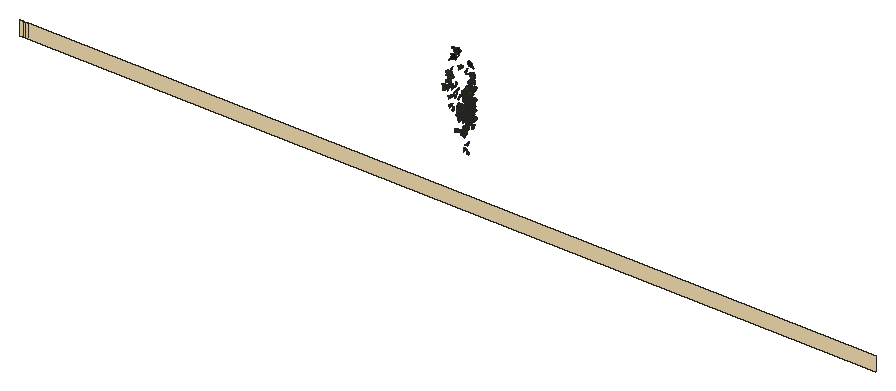
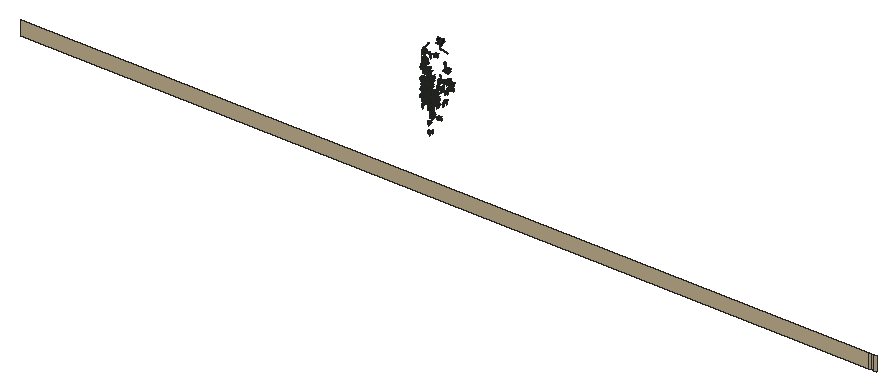
# SketchUp Ruby script. Lengths in inches.
U = 1.inch
M = Sketchup.active_model
def pt(a) = Geom::Point3d.new(a.map { |v| v * U })
def face(e, loops, mat)
  f = e.add_face(loops[0].map { |a| pt(a) })
  loops[1..].each { |l| e.add_face(l.map { |a| pt(a) }).erase! }
  f.material = f.back_material = mat if mat
  f
end
# faces: each face lists its corners as indices into pts; further lists are holes
def faces(e, pts, list, mat = nil) = list.each { |f| face(e, (f[0].is_a?(Array) ? f : [f]).map { |l| l.map { |i| pts[i] } }, mat) }
# xy, xz, yz: faces in a plane at the given z, y or x. An outline is a flat list of corners, or four numbers for a rectangle; further outlines are holes
def ring(l) = l.size == 4 ? [[l[0], l[1]], [l[2], l[1]], [l[2], l[3]], [l[0], l[3]]] : l.each_slice(2).to_a
def flat(e, list, mat, &to3) = list.each { |f| face(e, (f[0].is_a?(Array) ? f : [f]).map { |l| ring(l).map { |u, v| to3.(u, v) } }, mat) }
def xy(e, z, list, mat = nil) = flat(e, list, mat) { |x, y| [x, y, z] }
def xz(e, y, list, mat = nil) = flat(e, list, mat) { |x, z| [x, y, z] }
def yz(e, x, list, mat = nil) = flat(e, list, mat) { |y, z| [x, y, z] }
def lines(e, pts, list) = list.each { |a, b| e.add_line(pt(pts[a]), pt(pts[b])) }
# prism: a flat outline (further loops are holes) pulled along v
def prism(e, loops, v, mat = nil)
  f = face(e, loops, mat); d = Geom::Vector3d.new(v.map { |x| x * U })
  f.pushpull(f.normal.samedirection?(d) ? d.length : -d.length)
end
def box(e, o, s, mat = nil) = prism(e, [[o, [o[0] + s[0], o[1], o[2]], [o[0] + s[0], o[1] + s[1], o[2]], [o[0], o[1] + s[1], o[2]]]], [0, 0, s[2]], mat)
def at(x, y, z, deg = 0) = Geom::Transformation.translation(pt([x, y, z])) * Geom::Transformation.rotation(ORIGIN, Z_AXIS, deg.degrees)
def axes(o, x, y, z) = Geom::Transformation.new([*x, 0, *y, 0, *z, 0, *pt(o).to_a, 1])
def part(name) = M.definitions.add(name)
# library, detail: a bought-in or finely detailed component or shape, given as its bounding box
def library(name, o, s) = part(name).tap { |d| box(d.entities, o, s) }
def detail(e, o, s) = box(e.add_group.entities, o, s)
def put(e, d, t, mat = nil) = e.add_instance(d, t).tap { |i| i.material = mat if mat }
def group(e, t, mat = nil) = e.add_group.tap { |g| g.transformation = t; g.material = mat if mat }.entities
root = M.entities
M.materials.add("1026 AP 7946 SUNNY SIDE UP").color = [254, 231, 186]
M.materials.add("efeu1").color = [18, 25, 13]
M.materials.add("efeu2").color = [43, 57, 29]
c1 = part("ivyleaf_10")
p = [[0,0.5,-0.03],[-0.0625,2.02,-0.43],[-0.19,2.01,-0.46],[-0.54,1.05,-0.29],[-0.52,0.625,-0.18],[-0.83,0.76,-0.28],
  [-1.16,0.64,-0.33],[-1.15,0.33,-0.24],[-0.77,-0.39,0.02],[-0.3,-0.51,0.16],[0.04,-0.48,0.23],[-0.02,2.01,-0.4375],
  [-0.06,2.01,-0.43],[0.04,-0.49,0.23],[0.67,-0.49,0.14],[1.38,0.36,-0.2],[1.375,0.51,-0.24],[0.81,0.65,-0.19],
  [0.62,0.59,-0.15],[0.6,1.09,-0.28],[0.5,1.23,-0.31]]
faces(c1.entities,p,[[0,1,2,3,4,5,6,7,8,9,10],[11,12,0,13,14,15,16,17,18,19,20]],"efeu2")
c2 = part("ivyleaf_9")
p = [[1.54,2.16,1.25],[1.36,2.04,1.19],[-0.21,0.99,0.68],[-0.71,1.11,0.82],[-0.85,0.86,0.67],[-0.8,0.17,0.21],
  [-0.9,-0.01,0.1],[-0.67,-0.16,-0.02],[-0.08,-0.08,-0.05],[-0.03,-0.6,-0.4],[0.65,-0.88,-0.66],[0.83,-0.6,-0.49],
  [1.29,-0.42,-0.43],[1.8125,-0.07,-0.26],[1.21,0.44,0.15]]
faces(c2.entities,p,[[0,1,2,3,4,5,6,7,8,9,10,11,12,13,14]],"efeu1")
xz(root,213.1,[[29.49,246,29.75,248],[29.75,246,152.98,248]],"1026 AP 7946 SUNNY SIDE UP")
p = [[28.98,213.12,246],[28.98,213.12,248],[28.65,213.13,248],[28.65,213.13,246],[29.19,213.11,246],[29.19,213.11,248],
  [29.49,213.1,246],[29.49,213.1,248]]
faces(root,p,[[0,1,2,3],[4,5,1,0],[6,7,5,4]],"1026 AP 7946 SUNNY SIDE UP")
put(root,c1,axes([90.43,213.11,261.01],[0.21131,0.11138,-0.12925],[-0.15052,-0.08209,-0.18028],[-0.21754,0.16498,-0.00081]),"1026 AP 7946 SUNNY SIDE UP")
put(root,c1,axes([90.74,212.72,261.5625],[-0.28486,-0.07479,0.10189],[-0.1113,-0.08227,-0.1973],[0.16073,-0.18952,0.04395]),"1026 AP 7946 SUNNY SIDE UP")
put(root,c1,axes([90.68,213.08,261.15],[0.03809,0.2156,-0.007],[-0.00257,-0.00789,-0.22355],[-0.33923,0.02427,0.00091]),"1026 AP 7946 SUNNY SIDE UP")
put(root,c1,axes([90.82,213.05,262.11],[-0.11033,-0.17291,-0.12471],[0.18767,0.07159,-0.17763],[0.27267,-0.11923,0.0718]),"1026 AP 7946 SUNNY SIDE UP")
put(root,c1,axes([91.14,212.875,263.34],[0.33201,0.02527,-0.08737],[-0.12701,-0.03553,-0.2179],[-0.05739,0.22481,-0.02325]),"1026 AP 7946 SUNNY SIDE UP")
put(root,c1,axes([91.26,213,261.64],[-0.11322,-0.2058,0.02896],[-0.00445,-0.03002,-0.22467],[0.32683,-0.0717,0.00698]),"1026 AP 7946 SUNNY SIDE UP")
put(root,c1,axes([91.27,212.99,260.25],[-0.06266,-0.17143,0.12102],[0.02951,-0.12305,-0.1777],[0.32631,-0.02179,0.03931]),"1026 AP 7946 SUNNY SIDE UP")
put(root,c1,axes([91.35,213.01,259.1],[-0.02837,-0.19808,0.05526],[0.00033,-0.055,-0.20517],[0.32315,-0.01733,0.00506]),"1026 AP 7946 SUNNY SIDE UP")
put(root,c1,axes([91.35,212.87,262.98],[0.33522,0.0503,-0.06781],[-0.09987,-0.01866,-0.22574],[-0.08419,0.22242,-0.00223]),"1026 AP 7946 SUNNY SIDE UP")
put(root,c1,axes([91.45,212.98,263.93],[0.10871,-0.22409,0.02547],[0.00264,-0.02667,-0.24167],[0.35472,0.06887,-0.00601]),"1026 AP 7946 SUNNY SIDE UP")
put(root,c1,axes([91.64,212.99,261.61],[-0.10015,-0.2016,0.0619],[0.00589,-0.06504,-0.21697],[0.33123,-0.0598,0.02258]),"1026 AP 7946 SUNNY SIDE UP")
put(root,c1,axes([91.59,213,258.76],[0.05866,-0.19159,-0.06292],[0.04007,0.06504,-0.19729],[0.31313,0.02757,0.03704]),"1026 AP 7946 SUNNY SIDE UP")
put(root,c1,axes([91.74,213,260.67],[0.12014,-0.20112,-0.00474],[-0.00381,0.00278,-0.22162],[0.31627,0.07643,-0.00087]),"1026 AP 7946 SUNNY SIDE UP")
put(root,c2,axes([91.9,212.98,265.61],[-0.38272,0.01155,-0.00637],[0.00608,-0.04787,-0.24647],[-0.01974,-0.23873,0.04766]),"1026 AP 7946 SUNNY SIDE UP")
put(root,c1,axes([92.04,213.01,262.04],[0.13694,-0.18694,-0.08959],[-0.03553,0.08402,-0.21149],[0.32153,0.0889,0.01479]),"1026 AP 7946 SUNNY SIDE UP")
put(root,c1,axes([92.04,213,260.51],[0.04944,-0.20726,-0.04746],[-0.01887,0.04357,-0.21564],[0.33291,0.03325,-0.00517]),"1026 AP 7946 SUNNY SIDE UP")
put(root,c2,axes([92.06,212.86,266.8],[0.28129,0.11124,-0.138],[-0.16928,-0.08143,-0.21723],[-0.21616,0.20853,-0.00946]),"1026 AP 7946 SUNNY SIDE UP")
put(root,c1,axes([92.11,213,266.48],[0.29158,0.16408,-0.0095],[0.00728,-0.02051,-0.2545],[-0.25839,0.18458,-0.01789]),"1026 AP 7946 SUNNY SIDE UP")
put(root,c1,axes([92.31,213.01,261.42],[-0.04721,-0.21748,0.0158],[0.00085,-0.0168,-0.22625],[0.34295,-0.02989,0.00274]),"1026 AP 7946 SUNNY SIDE UP")
put(root,c2,axes([92.19,213.03,266.62],[0.03356,-0.24492,-0.01512],[-0.00555,0.01303,-0.25318],[0.38564,0.0215,-0.00232]),"1026 AP 7946 SUNNY SIDE UP")
put(root,c1,axes([92.39,213,258.31],[-0.10605,-0.19066,0.00425],[0.00501,-0.00665,-0.20831],[0.29986,-0.06732,0.00498]),"1026 AP 7946 SUNNY SIDE UP")
put(root,c1,axes([92.4375,213.01,259.21],[-0.02056,-0.20235,0.04331],[-0.00146,-0.04322,-0.20913],[0.32533,-0.01298,0.0018]),"1026 AP 7946 SUNNY SIDE UP")
put(root,c1,axes([92.56,212.68,256.39],[-0.19085,-0.09234,0.13648],[-0.11755,-0.11548,-0.15356],[0.22584,-0.13814,0.03541]),"1026 AP 7946 SUNNY SIDE UP")
put(root,c1,axes([92.54,213,260.57],[0.04857,-0.21234,-0.02038],[0.00425,0.01916,-0.22087],[0.33514,0.03053,0.00576]),"1026 AP 7946 SUNNY SIDE UP")
put(root,c1,axes([92.66,212.88,258.8],[-0.30872,-0.01749,0.05926],[-0.08792,-0.01994,-0.20265],[0.03512,-0.20364,0.01355]),"1026 AP 7946 SUNNY SIDE UP")
put(root,c1,axes([92.79,212.98,264.62],[-0.16114,-0.17711,0.12254],[-0.00933,-0.13061,-0.20464],[0.33622,-0.0885,0.05305]),"1026 AP 7946 SUNNY SIDE UP")
put(root,c1,axes([92.74,212.5,257.9],[-0.08186,0.18415,0.0993],[-0.04937,0.09017,-0.19655],[-0.3223,-0.06058,0.00489]),"1026 AP 7946 SUNNY SIDE UP")
put(root,c1,axes([92.62,212.85,258.92],[0.23234,-0.02625,0.14564],[0.21213,-0.04544,-0.15406],[0.07888,0.19949,-0.01468]),"1026 AP 7946 SUNNY SIDE UP")
put(root,c1,axes([92.85,212.99,259.37],[-0.13289,-0.16948,0.09],[-0.00219,-0.09603,-0.19176],[0.3005,-0.07565,0.03841]),"1026 AP 7946 SUNNY SIDE UP")
put(root,c1,axes([92.78,212.88,259.09],[-0.28995,0.0132,-0.09613],[0.14014,-0.04269,-0.18777],[-0.0485,-0.20224,0.03212]),"1026 AP 7946 SUNNY SIDE UP")
put(root,c1,axes([92.75,212.75,258.92],[0.31721,0.04987,0.0593],[0.09174,0.00232,-0.21375],[-0.07646,0.2097,-0.01045]),"1026 AP 7946 SUNNY SIDE UP")
put(root,c1,axes([93.05,212.73,259.75],[0.23814,-0.02438,-0.16367],[-0.25128,-0.00121,-0.15689],[0.02508,0.21939,-0.01775]),"1026 AP 7946 SUNNY SIDE UP")
put(root,c1,axes([93.02,212.68,258.34],[0.16766,-0.17255,-0.01512],[-0.03274,0.00319,-0.20829],[0.2702,0.10746,-0.01585]),"1026 AP 7946 SUNNY SIDE UP")
put(root,c1,axes([93.09,212.57,258.21],[-0.25147,0.09551,0.08344],[-0.11869,0.03021,-0.19135],[-0.15643,-0.17646,0.01104]),"1026 AP 7946 SUNNY SIDE UP")
put(root,c1,axes([93.09,212.68,258.49],[0.21871,-0.09967,-0.11551],[-0.12517,0.07967,-0.1751],[0.19916,0.15952,0.0168]),"1026 AP 7946 SUNNY SIDE UP")
put(root,c1,axes([93.15,212.77,258.625],[-0.11542,0.17134,0.08953],[-0.07992,0.07132,-0.19082],[-0.29061,-0.08766,0.01692]),"1026 AP 7946 SUNNY SIDE UP")
put(root,c1,axes([93.18,213,260.43],[-0.01833,0.21421,-0.01878],[-0.00009,-0.01948,-0.22111],[-0.33821,-0.0116,0.00107]),"1026 AP 7946 SUNNY SIDE UP")
put(root,c1,axes([93.09,212.7,258.11],[0.20077,0.12225,0.10831],[0.12065,0.07087,-0.18168],[-0.22217,0.14896,-0.00079]),"1026 AP 7946 SUNNY SIDE UP")
put(root,c1,axes([93.21,212.91,261.51],[0.0258,-0.14768,0.16948],[0.08976,-0.1574,-0.15158],[0.33685,0.05325,0.02741]),"1026 AP 7946 SUNNY SIDE UP")
put(root,c1,axes([93.34,212.62,256.24],[-0.16914,0.16875,-0.05533],[-0.03202,0.05176,0.20619],[0.27708,0.109,-0.00994]),"1026 AP 7946 SUNNY SIDE UP")
put(root,c1,axes([93.33,212.81,259.53],[-0.18979,-0.1549,0.07606],[-0.0211,-0.08251,-0.19906],[0.26959,-0.11551,0.03796]),"1026 AP 7946 SUNNY SIDE UP")
put(root,c1,axes([93.35,212.72,261.43],[0.13951,-0.18949,-0.09731],[-0.07996,0.07915,-0.21476],[0.3224,0.10163,-0.01116]),"1026 AP 7946 SUNNY SIDE UP")
put(root,c1,axes([93.29,212.96,257.89],[0.21052,0.1381,-0.06588],[-0.06715,-0.04874,-0.19841],[-0.23022,0.1405,-0.00237]),"1026 AP 7946 SUNNY SIDE UP")
put(root,c1,axes([93.34,212.95,259.24],[-0.2797,-0.1015,0.0425],[-0.00687,-0.07305,-0.20214],[0.17249,-0.1675,0.06087]),"1026 AP 7946 SUNNY SIDE UP")
put(root,c1,axes([93.26,212.92,260.7],[0.216,-0.16577,0.02402],[0.00205,0.03242,0.22086],[-0.26342,-0.13568,0.02141]),"1026 AP 7946 SUNNY SIDE UP")
put(root,c1,axes([93.34,212.98,258.15],[-0.21255,-0.15154,-0.01769],[0.03895,-0.00033,-0.20832],[0.23647,-0.13616,0.01841]),"1026 AP 7946 SUNNY SIDE UP")
put(root,c1,axes([93.41,212.6875,259.4375],[-0.26978,-0.12119,0.0086],[0.00422,-0.01942,-0.21577],[0.19105,-0.17071,0.01692]),"1026 AP 7946 SUNNY SIDE UP")
put(root,c1,axes([93.38,212.66,256.64],[-0.13831,-0.18167,-0.05645],[0.05848,0.04156,-0.20713],[0.2921,-0.09434,0.01474]),"1026 AP 7946 SUNNY SIDE UP")
put(root,c1,axes([93.45,212.98,261.09],[-0.13459,-0.19887,0.03309],[0.02143,-0.04174,-0.22133],[0.31632,-0.08179,0.02907]),"1026 AP 7946 SUNNY SIDE UP")
put(root,c1,axes([93.5,212.68,259.39],[0.15219,0.12868,-0.14001],[-0.14624,-0.10066,-0.16612],[-0.25636,0.13382,0.01164]),"1026 AP 7946 SUNNY SIDE UP")
put(root,c1,axes([93.46,212.875,260.84],[-0.06286,0.19099,0.09956],[-0.04698,0.09126,-0.20025],[-0.3325,-0.049,0.00947]),"1026 AP 7946 SUNNY SIDE UP")
put(root,c1,axes([93.51,212.99,261.25],[-0.17988,-0.1835,0.0419],[0.0137,-0.05393,-0.2201],[0.29558,-0.10917,0.0357]),"1026 AP 7946 SUNNY SIDE UP")
put(root,c1,axes([93.52,212.67,256.21],[-0.21052,-0.15891,0.0039],[0.01108,-0.01205,-0.21371],[0.24973,-0.13342,0.01277]),"1026 AP 7946 SUNNY SIDE UP")
put(root,c1,axes([93.5625,213.01,264.37],[0.07642,-0.23137,-0.00155],[-0.00368,-0.0003,-0.24354],[0.36378,0.0486,-0.00214]),"1026 AP 7946 SUNNY SIDE UP")
put(root,c1,axes([93.46,212.99,261.1],[0.26048,0.14171,0.02515],[0.04506,0.00271,-0.22392],[-0.22136,0.16731,-0.01599]),"1026 AP 7946 SUNNY SIDE UP")
put(root,c1,axes([93.55,213,261.39],[0.26969,0.13224,-0.04458],[-0.06567,-0.01783,-0.22292],[-0.20908,0.17617,0.01252]),"1026 AP 7946 SUNNY SIDE UP")
put(root,c1,axes([93.5,212.55,257.04],[-0.0052,-0.11033,-0.18527],[0.12626,0.16502,-0.10522],[0.30589,-0.06999,0.04028]),"1026 AP 7946 SUNNY SIDE UP")
put(root,c1,axes([93.58,212.52,254.21],[0.01807,-0.0674,-0.20159],[0.01767,0.19551,-0.06768],[0.32437,-0.0069,0.01491]),"1026 AP 7946 SUNNY SIDE UP")
put(root,c1,axes([93.41,212.6875,256.09],[0.05021,-0.05007,0.19931],[0.24977,-0.11299,-0.05771],[0.19138,0.1606,0.02303]),"1026 AP 7946 SUNNY SIDE UP")
put(root,c1,axes([93.625,212.74,261.33],[-0.15685,-0.20548,-0.01947],[0.0295,0.01057,-0.23491],[0.32296,-0.10076,0.01201]),"1026 AP 7946 SUNNY SIDE UP")
put(root,c1,axes([93.57,212.95,258.67],[-0.03543,0.19867,-0.05643],[0.00005,-0.05624,-0.20621],[-0.32452,-0.0217,0.00613]),"1026 AP 7946 SUNNY SIDE UP")
put(root,c1,axes([93.625,212.97,258.05],[0.20066,-0.1526,-0.04245],[-0.01011,0.0468,-0.20308],[0.24798,0.12539,0.02607]),"1026 AP 7946 SUNNY SIDE UP")
put(root,c1,axes([93.72,212.92,258.33],[-0.25929,-0.08689,0.08746],[-0.04461,-0.11236,-0.17489],[0.1863,-0.14785,0.07985]),"1026 AP 7946 SUNNY SIDE UP")
put(root,c1,axes([93.58,213,261.47],[-0.12564,-0.12532,-0.16994],[0.16969,0.12485,-0.15149],[0.27701,-0.13332,0.01572]),"1026 AP 7946 SUNNY SIDE UP")
put(root,c1,axes([93.79,212.96,259.05],[-0.16938,-0.13332,0.12401],[-0.0856,-0.11045,-0.17575],[0.27,-0.11865,0.02208]),"1026 AP 7946 SUNNY SIDE UP")
put(root,c1,axes([93.68,212.72,260.14],[-0.17667,-0.18099,-0.0282],[0.06659,0.00434,-0.21672],[0.27978,-0.11532,0.03377]),"1026 AP 7946 SUNNY SIDE UP")
put(root,c1,axes([93.7,212.91,259.41],[0.035,-0.18835,-0.0957],[0.04289,0.09417,-0.19161],[0.32668,0.00782,0.03541]),"1026 AP 7946 SUNNY SIDE UP")
put(root,c1,axes([93.66,212.95,258.82],[0.01118,0.20606,-0.03149],[-0.00066,-0.03174,-0.21259],[-0.32782,0.00709,-0.00065]),"1026 AP 7946 SUNNY SIDE UP")
put(root,c1,axes([93.74,212.68,256.65],[0.19108,-0.16089,-0.04959],[-0.03727,0.04125,-0.20738],[0.261,0.12367,0.00669]),"1026 AP 7946 SUNNY SIDE UP")
put(root,c1,axes([93.75,212.73,256.34],[0.02724,-0.1933,0.06967],[0.00259,-0.06884,-0.20029],[0.32257,0.01687,-0.00427]),"1026 AP 7946 SUNNY SIDE UP")
put(root,c1,axes([93.67,212.74,261.93],[-0.00855,-0.20428,0.11303],[0.18292,-0.09841,-0.18148],[0.3164,0.05137,0.10797]),"1026 AP 7946 SUNNY SIDE UP")
put(root,c1,axes([93.77,212.95,259.08],[0.00274,-0.14114,0.15974],[0.04699,-0.15412,-0.14502],[0.32727,0.02331,0.01948]),"1026 AP 7946 SUNNY SIDE UP")
put(root,c1,axes([93.82,212.95,260.29],[0.17215,-0.17892,-0.05197],[-0.02637,0.04762,-0.21556],[0.29069,0.11028,0.01122]),"1026 AP 7946 SUNNY SIDE UP")
put(root,c1,axes([93.7,212.66,257.28],[-0.27301,-0.05989,-0.11254],[0.17033,0.01877,-0.18846],[0.09577,-0.20409,0.01438]),"1026 AP 7946 SUNNY SIDE UP")
put(root,c1,axes([93.84,212.95,258.95],[0.05924,-0.20543,-0.0107],[-0.00022,0.00935,-0.2151],[0.32335,0.03764,0.00181]),"1026 AP 7946 SUNNY SIDE UP")
put(root,c1,axes([93.82,212.75,260.42],[-0.10429,-0.195,-0.06749],[0.05532,0.05589,-0.21132],[0.31813,-0.07364,0.01463]),"1026 AP 7946 SUNNY SIDE UP")
put(root,c1,axes([93.86,212.96,261.5],[0.00883,-0.22032,0.02496],[-0.00096,-0.0255,-0.22719],[0.34874,0.00551,-0.00126]),"1026 AP 7946 SUNNY SIDE UP")
put(root,c1,axes([93.59,212.96,258.7],[0.11424,0.05307,0.19332],[0.2747,0.07056,-0.08997],[-0.13524,0.18815,-0.01944]),"1026 AP 7946 SUNNY SIDE UP")
put(root,c1,axes([93.97,212.63,254.06],[-0.22714,0.11155,0.09929],[-0.14575,0.03508,-0.18596],[-0.17942,-0.16972,0.02536]),"1026 AP 7946 SUNNY SIDE UP")
put(root,c1,axes([93.86,212.83,261.08],[-0.35723,0.03082,-0.02764],[0.03697,-0.02656,-0.23516],[-0.05277,-0.22724,0.02236]),"1026 AP 7946 SUNNY SIDE UP")
put(root,c1,axes([93.85,212.72,260.53],[-0.30756,0.08587,-0.03911],[0.04209,-0.03425,-0.21927],[-0.14182,-0.19638,0.01974]),"1026 AP 7946 SUNNY SIDE UP")
put(root,c1,axes([94.1,212.78,260.9],[0.20007,-0.04126,-0.17832],[-0.27108,0.02293,-0.13624],[0.06781,0.21341,-0.01853]),"1026 AP 7946 SUNNY SIDE UP")
put(root,c1,axes([94.03,212.92,260.6],[-0.02069,-0.20849,0.06151],[-0.0073,-0.06072,-0.21556],[0.34144,-0.01393,-0.00088]),"1026 AP 7946 SUNNY SIDE UP")
put(root,c1,axes([94.02,212.95,259.65],[-0.09963,-0.20392,-0.01393],[0.00663,0.01164,-0.21992],[0.32117,-0.0635,0.00022]),"1026 AP 7946 SUNNY SIDE UP")
put(root,c1,axes([94.04,212.95,259.36],[-0.0644,-0.20786,0.00153],[0.00268,-0.00305,-0.21826],[0.32686,-0.04093,0.00209]),"1026 AP 7946 SUNNY SIDE UP")
put(root,c1,axes([94.04,212.88,260.8],[-0.3429,-0.0134,-0.00028],[0.00235,-0.02111,-0.22415],[0.02094,-0.21705,0.02053]),"1026 AP 7946 SUNNY SIDE UP")
put(root,c1,axes([94.04,212.62,257.82],[-0.05097,-0.18416,-0.10778],[0.02682,0.10216,-0.19204],[0.33114,-0.03662,-0.00103]),"1026 AP 7946 SUNNY SIDE UP")
put(root,c1,axes([93.9,212.99,262.32],[-0.27207,-0.03081,-0.14718],[0.22527,-0.07834,-0.16199],[-0.04409,-0.21014,0.08055]),"1026 AP 7946 SUNNY SIDE UP")
put(root,c1,axes([94.08,212.55,255.21],[-0.08192,-0.18683,-0.06316],[0.02876,0.05744,-0.19947],[0.30733,-0.05518,0.00183]),"1026 AP 7946 SUNNY SIDE UP")
put(root,c1,axes([94.22,212.72,258.32],[0.20303,-0.02272,-0.16374],[-0.22201,0.0807,-0.12969],[0.11977,0.1881,0.03718]),"1026 AP 7946 SUNNY SIDE UP")
put(root,c1,axes([94.14,212.95,262.16],[0.04081,-0.14407,-0.17869],[-0.02159,0.17244,-0.14937],[0.3529,0.02721,0.01153]),"1026 AP 7946 SUNNY SIDE UP")
put(root,c1,axes([94.1,212.96,259.73],[0.03214,0.15247,0.15446],[-0.0459,0.15034,-0.15341],[-0.33212,-0.00603,0.03615]),"1026 AP 7946 SUNNY SIDE UP")
put(root,c1,axes([94.02,212.72,262.375],[0.2486,0.17185,0.0332],[0.04789,0.01438,-0.24013],[-0.27043,0.16052,-0.01201]),"1026 AP 7946 SUNNY SIDE UP")
put(root,c1,axes([94.14,212.85,258.65],[0.13999,-0.19496,0.02421],[0.00372,-0.02595,-0.22077],[0.30896,0.08865,-0.00831]),"1026 AP 7946 SUNNY SIDE UP")
put(root,c1,axes([94.03,212.875,258.03],[0.32265,0.00172,0.05758],[0.08758,-0.02466,-0.21006],[0.0076,0.21124,-0.02374]),"1026 AP 7946 SUNNY SIDE UP")
put(root,c2,axes([93.97,212.96,265.47],[0.2147,-0.1884,-0.07224],[-0.03993,0.06663,-0.23861],[0.31298,0.13774,0.01912]),"1026 AP 7946 SUNNY SIDE UP")
put(root,c1,axes([93.96,212.66,258.07],[0.22436,0.0212,0.16766],[0.24564,0.04805,-0.14737],[-0.07849,0.21094,0.01803]),"1026 AP 7946 SUNNY SIDE UP")
put(root,c1,axes([94.23,212.73,260.875],[-0.08566,-0.22081,-0.0432],[0.04754,0.03426,-0.23312],[0.34984,-0.05872,0.0211]),"1026 AP 7946 SUNNY SIDE UP")
put(root,c1,axes([94.2,212.79,263.06],[0.03965,0.2271,0.03263],[-0.00991,0.03124,-0.235],[-0.36013,0.02415,0.01006]),"1026 AP 7946 SUNNY SIDE UP")
put(root,c1,axes([94.22,212.79,262.93],[-0.15941,0.20488,-0.02298],[0.00226,-0.02545,-0.23542],[-0.32425,-0.1009,0.00966]),"1026 AP 7946 SUNNY SIDE UP")
put(root,c1,axes([94.31,212.95,260.26],[0.22196,0.10175,-0.13428],[-0.15408,-0.0875,-0.17942],[-0.21032,0.17149,-0.01026]),"1026 AP 7946 SUNNY SIDE UP")
put(root,c1,axes([94.16,212.78,260.96],[-0.15295,-0.15544,-0.14582],[0.18234,0.08929,-0.18374],[0.27462,-0.14586,0.04078]),"1026 AP 7946 SUNNY SIDE UP")
put(root,c1,axes([94.3125,212.95,260.3],[-0.02308,-0.21657,-0.02028],[0.00534,0.01827,-0.2235],[0.34173,-0.01491,0.00212]),"1026 AP 7946 SUNNY SIDE UP")
put(root,c1,axes([94.28,212.63,260.875],[-0.33544,-0.04485,-0.04404],[0.07256,-0.01409,-0.22342],[0.0646,-0.21707,0.02228]),"1026 AP 7946 SUNNY SIDE UP")
put(root,c1,axes([94.25,212.97,263.13],[0.3389,0.08237,0.00802],[0.02123,-0.01491,-0.237],[-0.12829,0.21514,-0.01804]),"1026 AP 7946 SUNNY SIDE UP")
put(root,c1,axes([94.36,212.9375,258.2],[-0.03504,-0.20174,0.02816],[0.00244,-0.02882,-0.20921],[0.32035,-0.02185,0.00467]),"1026 AP 7946 SUNNY SIDE UP")
put(root,c1,axes([94.47,212.74,261.7],[-0.1616,-0.08681,0.19879],[-0.11005,-0.18905,-0.1268],[0.31472,-0.11067,0.05773]),"1026 AP 7946 SUNNY SIDE UP")
put(root,c1,axes([94.12,212.78,258.89],[0.17718,-0.04541,0.18398],[0.27898,-0.03088,-0.12342],[0.07967,0.20911,0.02304]),"1026 AP 7946 SUNNY SIDE UP")
put(root,c1,axes([94.41,212.93,258.4],[-0.06044,-0.18733,0.07688],[-0.02228,-0.07435,-0.19744],[0.3169,-0.04095,0.00078]),"1026 AP 7946 SUNNY SIDE UP")
put(root,c1,axes([94.34,212.98,262.21],[-0.34609,-0.0276,-0.05116],[0.08102,-0.01481,-0.22762],[0.0371,-0.22511,0.0199]),"1026 AP 7946 SUNNY SIDE UP")
put(root,c1,axes([94.43,212.93,260.02],[-0.18459,-0.17734,0.03584],[-0.01366,-0.0371,-0.2189],[0.28415,-0.11699,0.01276]),"1026 AP 7946 SUNNY SIDE UP")
put(root,c1,axes([94.38,212.95,259.97],[0.20826,-0.16686,-0.0348],[0.00313,0.04314,-0.2173],[0.26738,0.12946,0.02965]),"1026 AP 7946 SUNNY SIDE UP")
put(root,c1,axes([94.45,212.95,258.18],[0.20452,-0.14874,-0.0889],[-0.05437,0.0823,-0.20132],[0.26418,0.13208,0.02739]),"1026 AP 7946 SUNNY SIDE UP")
put(root,c1,axes([94.42,212.8,259.43],[0.3399,-0.02835,-0.03148],[-0.05068,-0.01266,-0.22402],[0.04127,0.21792,-0.01581]),"1026 AP 7946 SUNNY SIDE UP")
put(root,c1,axes([94.33,212.62,258.88],[0.00605,0.03126,0.22693],[0.08466,0.21345,-0.03096],[-0.33915,0.05384,-0.00368]),"1026 AP 7946 SUNNY SIDE UP")
put(root,c1,axes([94.52,212.8125,263.85],[0.24856,-0.15806,-0.07616],[-0.10199,0.03808,-0.22932],[0.25407,0.16991,-0.01755]),"1026 AP 7946 SUNNY SIDE UP")
put(root,c1,axes([94.5,212.98,259.06],[-0.02983,-0.20772,0.01267],[-0.00461,-0.01326,-0.21495],[0.32727,-0.01912,-0.00187]),"1026 AP 7946 SUNNY SIDE UP")
put(root,c1,axes([94.49,212.95,260.09],[0.13477,-0.19496,-0.04147],[-0.00195,0.0421,-0.21856],[0.31266,0.0843,0.01651]),"1026 AP 7946 SUNNY SIDE UP")
put(root,c1,axes([94.75,212.68,264.32],[0.04868,0.01132,-0.25206],[-0.38088,-0.03561,-0.03347],[-0.05782,0.24411,0.00827]),"1026 AP 7946 SUNNY SIDE UP")
put(root,c1,axes([94.46,212.94,260.58],[-0.04036,0.2152,-0.03453],[0.00095,-0.03491,-0.22345],[-0.34277,-0.02544,0.00345]),"1026 AP 7946 SUNNY SIDE UP")
put(root,c1,axes([94.54,212.96,260.47],[0.15243,-0.18285,-0.07252],[0.00007,0.07743,-0.20978],[0.3075,0.09062,0.036]),"1026 AP 7946 SUNNY SIDE UP")
put(root,c1,axes([94.57,212.9,259.68],[-0.14194,-0.18539,0.0557],[0.0045,-0.0621,-0.21071],[0.30408,-0.08562,0.02912]),"1026 AP 7946 SUNNY SIDE UP")
put(root,c1,axes([94.59,212.74,258.1875],[0.09213,-0.19593,-0.05651],[-0.01592,0.05304,-0.2103],[0.31907,0.05922,0.00582]),"1026 AP 7946 SUNNY SIDE UP")
put(root,c1,axes([94.61,212.88,258.24],[-0.14282,-0.15945,0.09275],[-0.01022,-0.0986,-0.18538],[0.28845,-0.08244,0.03936]),"1026 AP 7946 SUNNY SIDE UP")
put(root,c1,axes([94.6,212.94,260.19],[-0.10104,-0.20648,0.0089],[0.00705,-0.01167,-0.2227],[0.32496,-0.06395,0.0076]),"1026 AP 7946 SUNNY SIDE UP")
put(root,c1,axes([94.64,212.98,258.53],[-0.0243,-0.19808,0.05296],[-0.00795,-0.0523,-0.20498],[0.32212,-0.01623,-0.00106]),"1026 AP 7946 SUNNY SIDE UP")
put(root,c1,axes([94.47,212.68,263.42],[-0.28393,-0.05914,-0.15548],[0.24378,0.00123,-0.19201],[0.07269,-0.23512,0.03664]),"1026 AP 7946 SUNNY SIDE UP")
put(root,c1,axes([94.65,212.97,257.4375],[0.04566,-0.19446,-0.08075],[0.02404,0.07979,-0.20044],[0.32816,0.02121,0.02592]),"1026 AP 7946 SUNNY SIDE UP")
put(root,c1,axes([94.7,212.94,260.82],[-0.18736,-0.17675,0.05727],[-0.0016,-0.06663,-0.21698],[0.29182,-0.11385,0.03558]),"1026 AP 7946 SUNNY SIDE UP")
put(root,c1,axes([94.73,212.92,259.625],[-0.21019,-0.15365,0.06414],[-0.01711,-0.07276,-0.20659],[0.26064,-0.12869,0.03816]),"1026 AP 7946 SUNNY SIDE UP")
put(root,c1,axes([94.73,212.93,262.56],[-0.20181,-0.18404,0.04487],[-0.00688,-0.05099,-0.23],[0.29769,-0.12594,0.02511]),"1026 AP 7946 SUNNY SIDE UP")
put(root,c1,axes([94.68,212.93,259.18],[0.08896,-0.19017,-0.07283],[0.02614,0.0764,-0.20064],[0.31736,0.04702,0.03695]),"1026 AP 7946 SUNNY SIDE UP")
put(root,c1,axes([94.66,212.74,259.18],[-0.07137,0.18033,-0.10564],[0.00142,-0.10583,-0.19087],[-0.32699,-0.03982,0.02222]),"1026 AP 7946 SUNNY SIDE UP")
put(root,c1,axes([94.77,212.79,260.12],[-0.13481,-0.16102,0.11723],[-0.03266,-0.117,-0.18588],[0.30915,-0.08258,0.03148]),"1026 AP 7946 SUNNY SIDE UP")
put(root,c1,axes([94.71,212.69,257.65],[0.10854,-0.1842,0.04848],[0.0177,-0.04713,-0.20283],[0.29882,0.0697,-0.00559]),"1026 AP 7946 SUNNY SIDE UP")
put(root,c1,axes([94.81,212.95,258.66],[-0.2493,-0.11358,0.07259],[-0.03023,-0.08973,-0.19235],[0.20852,-0.1488,0.0589]),"1026 AP 7946 SUNNY SIDE UP")
put(root,c1,axes([94.72,212.95,261.01],[-0.23532,-0.16472,-0.01016],[0.09766,-0.0451,-0.21567],[0.24031,-0.14298,0.0777]),"1026 AP 7946 SUNNY SIDE UP")
put(root,c1,axes([94.77,212.89,258.875],[0.0845,-0.17923,0.09409],[0.02353,-0.09177,-0.19298],[0.31616,0.05474,-0.01078]),"1026 AP 7946 SUNNY SIDE UP")
put(root,c1,axes([94.79,212.78,264.34],[-0.19571,0.20172,0.01878],[-0.02041,0.01207,-0.24406],[-0.31766,-0.12505,0.00411]),"1026 AP 7946 SUNNY SIDE UP")
